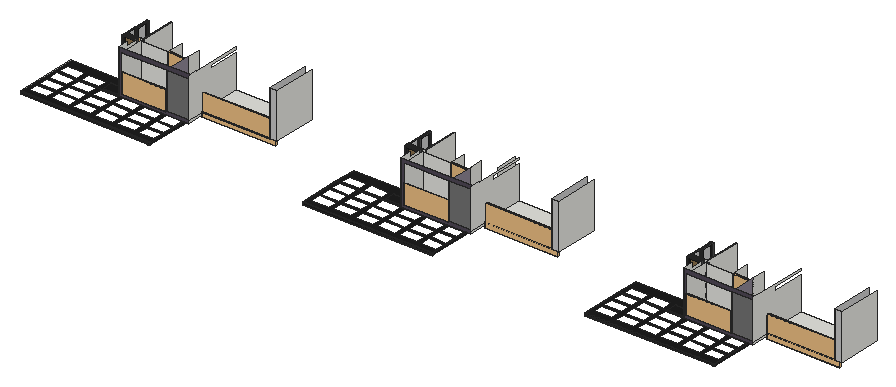
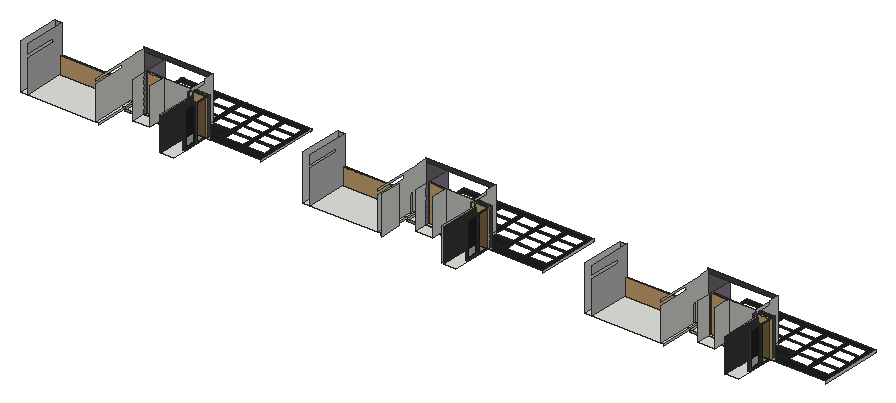
# SketchUp Ruby script. Lengths in inches.
U = 1.inch
M = Sketchup.active_model
def pt(a) = Geom::Point3d.new(a.map { |v| v * U })
def face(e, loops, mat)
  f = e.add_face(loops[0].map { |a| pt(a) })
  loops[1..].each { |l| e.add_face(l.map { |a| pt(a) }).erase! }
  f.material = f.back_material = mat if mat
  f
end
# faces: each face lists its corners as indices into pts; further lists are holes
def faces(e, pts, list, mat = nil) = list.each { |f| face(e, (f[0].is_a?(Array) ? f : [f]).map { |l| l.map { |i| pts[i] } }, mat) }
# xy, xz, yz: faces in a plane at the given z, y or x. An outline is a flat list of corners, or four numbers for a rectangle; further outlines are holes
def ring(l) = l.size == 4 ? [[l[0], l[1]], [l[2], l[1]], [l[2], l[3]], [l[0], l[3]]] : l.each_slice(2).to_a
def flat(e, list, mat, &to3) = list.each { |f| face(e, (f[0].is_a?(Array) ? f : [f]).map { |l| ring(l).map { |u, v| to3.(u, v) } }, mat) }
def xy(e, z, list, mat = nil) = flat(e, list, mat) { |x, y| [x, y, z] }
def xz(e, y, list, mat = nil) = flat(e, list, mat) { |x, z| [x, y, z] }
def yz(e, x, list, mat = nil) = flat(e, list, mat) { |y, z| [x, y, z] }
def lines(e, pts, list) = list.each { |a, b| e.add_line(pt(pts[a]), pt(pts[b])) }
# prism: a flat outline (further loops are holes) pulled along v
def prism(e, loops, v, mat = nil)
  f = face(e, loops, mat); d = Geom::Vector3d.new(v.map { |x| x * U })
  f.pushpull(f.normal.samedirection?(d) ? d.length : -d.length)
end
def box(e, o, s, mat = nil) = prism(e, [[o, [o[0] + s[0], o[1], o[2]], [o[0] + s[0], o[1] + s[1], o[2]], [o[0], o[1] + s[1], o[2]]]], [0, 0, s[2]], mat)
def at(x, y, z, deg = 0) = Geom::Transformation.translation(pt([x, y, z])) * Geom::Transformation.rotation(ORIGIN, Z_AXIS, deg.degrees)
def axes(o, x, y, z) = Geom::Transformation.new([*x, 0, *y, 0, *z, 0, *pt(o).to_a, 1])
def part(name) = M.definitions.add(name)
# library, detail: a bought-in or finely detailed component or shape, given as its bounding box
def library(name, o, s) = part(name).tap { |d| box(d.entities, o, s) }
def detail(e, o, s) = box(e.add_group.entities, o, s)
def put(e, d, t, mat = nil) = e.add_instance(d, t).tap { |i| i.material = mat if mat }
def group(e, t, mat = nil) = e.add_group.tap { |g| g.transformation = t; g.material = mat if mat }.entities
root = M.entities
M.materials.add("Glass_Tinted_Gray").color = [0, 0, 0]
M.materials["Glass_Tinted_Gray"].alpha = 0.125
M.materials.add("[0135_DarkGray]").color = [81, 81, 81]
M.materials.add("[Color M02]").color = [198, 198, 198]
M.materials.add("[Color M04]").color = [60, 133, 34]
M.materials.add("[Color M05]1").color = [114, 114, 114]
M.materials.add("[Color M06]").color = [79, 71, 84]
M.materials.add("[Color M07]").color = [58, 58, 58]
M.materials.add("[Color M08]").color = [30, 30, 30]
M.materials.add("[Formica Graystone]1").color = [140, 132, 147]
M.materials.add("[Mirror 02]").color = [229, 229, 229]
c1 = part("glass-railing")
detail(c1.entities,[0,0,0],[1.26,75.59,33.1875])
c2 = library("Sliding Gate",[0,0,0],[194.88,4.13,70.58])
c3 = part("PENTEK_RP Fineline 50S_SlidingDoor_Glass")
box(c3.entities,[0,0,0],[46.58,0.16,94.39],"Glass_Tinted_Gray")
c4 = part("PENTEK_RP Fineline 50S_SlidingDoor_GlazingBead")
box(c4.entities,[0,0,0],[45.47,0.59,0.56],"[0135_DarkGray]")
c5 = part("PENTEK_RP Fineline 50S_SlidingDoor_GlazingBead_2")
box(c5.entities,[0,0,0],[0.56,0.59,94.39],"[0135_DarkGray]")
c6 = part("PENTEK_RP Fineline 50S_SlidingDoor_Leaf_E1")
xy(c6.entities,0,[[0,0,0.93,1.97],[0.93,1.57,1.49,1.97]],"[0135_DarkGray]")
xy(c6.entities,96.25,[[0,0,0.93,0,0.93,1.57,1.49,1.57,1.49,1.97,0,1.97]],"[0135_DarkGray]")
xz(c6.entities,0,[[0,0,0.93,96.25]],"[0135_DarkGray]")
xz(c6.entities,1.57,[[0.93,0,1.49,95.32],[0.93,95.32,1.49,96.25]],"[0135_DarkGray]")
xz(c6.entities,1.97,[[0,0,1.49,96.25]],"[0135_DarkGray]")
yz(c6.entities,0,[[0,0,1.97,96.25]],"[0135_DarkGray]")
yz(c6.entities,0.93,[[0,0,1.57,0.93],[0,0.93,1.57,95.32],[0,95.32,1.57,96.25]],"[0135_DarkGray]")
yz(c6.entities,1.49,[[1.57,0,1.97,95.32],[1.57,95.32,1.97,96.25]],"[0135_DarkGray]")
c7 = part("PENTEK_RP Fineline 50S_SlidingDoor_Leaf_E2")
xy(c7.entities,0,[[0,0,0,1.57,0.56,1.57,0.56,1.97,46.02,1.97,46.02,1.57,46.58,1.57,46.58,0]],"[0135_DarkGray]")
xy(c7.entities,0.93,[[0,0,46.58,1.57]],"[0135_DarkGray]")
xy(c7.entities,1.49,[[0.56,1.57,46.02,1.97]],"[0135_DarkGray]")
xz(c7.entities,0,[[0,0,46.58,0.93]],"[0135_DarkGray]")
xz(c7.entities,1.57,[[0,0,0.56,0.93],[46.02,0,46.58,0.93],[0.56,0.93,46.02,1.49]],"[0135_DarkGray]")
xz(c7.entities,1.97,[[0.56,0,46.02,1.49]],"[0135_DarkGray]")
yz(c7.entities,0,[[0,0,1.57,0.93]],"[0135_DarkGray]")
yz(c7.entities,0.56,[[1.57,0,1.97,0.93],[1.57,0.93,1.97,1.49]],"[0135_DarkGray]")
yz(c7.entities,46.02,[[1.57,0,1.97,0.93],[1.57,0.93,1.97,1.49]],"[0135_DarkGray]")
yz(c7.entities,46.58,[[0,0,1.57,0.93]],"[0135_DarkGray]")
c8 = part("PENTEK_RP Fineline 50S_SlidingDoor_Leaf2")
put(c8.entities,c3,at(1.49,1.42,0.93))
put(c8.entities,c4,at(1.49,0,94.77))
put(c8.entities,c5,at(46.96,0,0.93))
put(c8.entities,c3,at(1.49,0.59,0.93),"[Mirror 02]")
put(c8.entities,c5,at(0.93,0,0.93))
put(c8.entities,c6,at(0,0,0))
put(c8.entities,c6,axes([48.44,0,0],[-1,0,0],[0,1,0],[0,0,1]))
put(c8.entities,c4,at(1.49,0,0.93))
put(c8.entities,c7,axes([0.93,0,96.25],[1,0,0],[0,1,0],[0,0,-1]))
put(c8.entities,c7,at(0.93,0,0))
c9 = library("Aluprof_MB-86_Drzwi_panelowe_003_S-0452",[0,0,0],[44.84,5.36,87])
c10 = library("Group\#1",[0,0,0],[29.75,5.78,110.95])
xy(root,117.06,[[264.14,305.5,671.22,306.625],[1150.61,305.5,1557.68,306.625],[2037.07,305.5,2444.15,306.625],[670.9,306.625,671.22,487.3125],[1557.37,306.625,1557.68,487.3125],
  [2443.83,306.625,2444.15,487.3125]])
xy(root,123.92,[[618.43,305.5,671.22,306.625],[1504.89,305.5,1557.68,306.625],[2391.36,305.5,2444.15,306.625],[670.9,306.625,671.22,487.3125],[1557.37,306.625,1557.68,487.3125],
  [2443.83,306.625,2444.15,487.3125]])
xy(root,123.92,[[264.14,305.5,473.73,306.625],[473.73,305.5,618.43,306.625],[1150.61,305.5,1360.2,306.625],[1360.2,305.5,1504.89,306.625],[2037.07,305.5,2246.66,306.625],
  [2246.66,305.5,2391.36,306.625]],"[Color M08]")
xy(root,125.0625,[[468.02,437.0625,468.02,441.875,470.84,441.875,470.84,475.3125,468.02,475.3125,468.02,521.5625,473.73,521.5625,473.73,437.0625],[[473.73,437.0625,618.43,521.5625],[481.77,441.875,539.73,475.3125],[550.67,442.1875,608.63,475.3125]],[[618.43,437.0625,618.43,521.5625,677.53,521.5625,677.53,487.3125,671.22,487.3125,671.22,437.0625],[619.57,441.86,669.03,475.3125]],[671.22,437.0625,686.84,487.3125],[1354.48,437.0625,1354.48,441.875,1357.3,441.875,1357.3,475.3125,1354.48,475.3125,1354.48,521.5625,1360.2,521.5625,1360.2,437.0625],
  [[1360.2,437.0625,1504.89,521.5625],[1368.24,441.875,1426.2,475.3125],[1437.14,442.1875,1495.1,475.3125]],[[1504.89,437.0625,1504.89,521.5625,1563.99,521.5625,1563.99,487.3125,1557.68,487.3125,1557.68,437.0625],[1506.03,441.86,1555.49,475.3125]],[1557.68,437.0625,1573.31,487.3125],[2240.94,437.0625,2240.94,441.875,2243.76,441.875,2243.76,475.3125,2240.94,475.3125,2240.94,521.5625,2246.66,521.5625,2246.66,437.0625],[[2246.66,437.0625,2391.36,521.5625],[2254.7,441.875,2312.66,475.3125],[2323.6,442.1875,2381.56,475.3125]],
  [[2391.36,437.0625,2391.36,521.5625,2450.46,521.5625,2450.46,487.3125,2444.15,487.3125,2444.15,437.0625],[2392.5,441.86,2441.96,475.3125]],[2444.15,437.0625,2459.77,487.3125],[468.02,441.875,470.84,475.3125],[1354.48,441.875,1357.3,475.3125],[2240.94,441.875,2243.76,475.3125]])
xy(root,125.0625,[[[264.14,305.5,671.22,437.0625],[412.875,401.625,470.84,435.86],[481.77,401.625,539.73,435.86],[343.98,401.625,401.9375,435.86],[550.67,401.75,608.63,435.86],[412.875,362.375,470.84,396.41],[481.77,362.375,539.73,396.41],[343.98,362.375,401.9375,396.41],[275.89,401.625,333.04,435.86],[275.89,362.375,333.04,396.41],[550.67,362.875,608.63,396.41],[412.875,323.5,470.84,356.95],[481.77,323.5,539.73,356.95],[550.67,323.5,608.63,356.95],[343.98,323.5,401.9375,356.95],[275.89,323.5,333.04,356.95],[619.57,402.41,669.03,435.86],[619.57,362.95,669.03,396.41],[619.57,323.5,669.03,356.95]],[[1150.61,305.5,1557.68,437.0625],[1368.24,401.625,1426.2,435.86],[1230.44,401.625,1288.4,435.86],[1299.34,401.625,1357.3,435.86],[1437.14,401.75,1495.1,435.86],[1368.24,362.375,1426.2,396.41],[1230.44,362.375,1288.4,396.41],[1299.34,362.375,1357.3,396.41],[1162.36,401.625,1219.5,435.86],[1162.36,362.375,1219.5,396.41],[1437.14,362.875,1495.1,396.41],[1368.24,323.5,1426.2,356.95],[1437.14,323.5,1495.1,356.95],[1230.44,323.5,1288.4,356.95],[1299.34,323.5,1357.3,356.95],[1162.36,323.5,1219.5,356.95],[1506.03,402.41,1555.49,435.86],[1506.03,362.95,1555.49,396.41],[1506.03,323.5,1555.49,356.95]],[[2037.07,305.5,2444.15,437.0625],[2185.8,401.625,2243.76,435.86],[2254.7,401.625,2312.66,435.86],[2116.91,401.625,2174.87,435.86],[2323.6,401.75,2381.56,435.86],[2185.8,362.375,2243.76,396.41],[2254.7,362.375,2312.66,396.41],[2116.91,362.375,2174.87,396.41],[2048.82,401.625,2105.97,435.86],[2048.82,362.375,2105.97,396.41],[2323.6,362.875,2381.56,396.41],[2185.8,323.5,2243.76,356.95],[2254.7,323.5,2312.66,356.95],[2323.6,323.5,2381.56,356.95],[2116.91,323.5,2174.87,356.95],[2048.82,323.5,2105.97,356.95],[2392.5,402.41,2441.96,435.86],[2392.5,362.95,2441.96,396.41],[2392.5,323.5,2441.96,356.95]],[[264.14,437.0625,468.02,437.0625,468.02,441.875,412.875,441.875,412.875,475.3125,468.02,475.3125,468.02,505.3125,264.14,505.3125],[343.98,441.875,401.9375,475.3125],[275.89,441.875,333.04,475.3125]],[[1150.61,437.0625,1354.48,437.0625,1354.48,441.875,1299.34,441.875,1299.34,475.3125,1354.48,475.3125,1354.48,505.3125,1150.61,505.3125],[1230.44,441.875,1288.4,475.3125],[1162.36,441.875,1219.5,475.3125]],
  [[2037.07,437.0625,2240.94,437.0625,2240.94,441.875,2185.8,441.875,2185.8,475.3125,2240.94,475.3125,2240.94,505.3125,2037.07,505.3125],[2116.91,441.875,2174.87,475.3125],[2048.82,441.875,2105.97,475.3125]],[412.875,441.875,468.02,475.3125],[1299.34,441.875,1354.48,475.3125],[2185.8,441.875,2240.94,475.3125]],"[Color M08]")
xy(root,131.0625,[[435.78,561.375,446.59,562.32],[1322.24,561.375,1333.06,562.32],[2208.71,561.375,2219.52,562.32]])
xy(root,135.875,[[478.55,437.0625,618.43,437.0625,618.43,521.5625,565.03,521.5625,565.03,509.6875,478.55,509.6875],[1365.01,437.0625,1504.89,437.0625,1504.89,521.5625,1451.49,521.5625,1451.49,509.6875,1365.01,509.6875],[2251.48,437.0625,2391.36,437.0625,2391.36,521.5625,2337.96,521.5625,2337.96,509.6875,2251.48,509.6875],[478.55,509.6875,565.03,521.5625],[1365.01,509.6875,1451.49,521.5625],
  [2251.48,509.6875,2337.96,521.5625],[565.03,521.5625,618.43,562.32],[1451.49,521.5625,1504.89,562.32],[2337.96,521.5625,2391.36,562.32]])
xy(root,136.125,[[677.53,487.3125,686.84,521.5625],[686.84,487.3125,901.22,623.84],[901.22,487.3125,923.77,623.84],[1563.99,487.3125,1573.31,521.5625],[1573.31,487.3125,1787.6875,623.84],
  [1787.6875,487.3125,1810.23,623.84],[2450.46,487.3125,2459.77,521.5625],[2459.77,487.3125,2674.15,623.84],[2674.15,487.3125,2696.7,623.84],[424.39,505.3125,463.64,646.3125],
  [463.64,505.3125,468.02,562.32],[1310.86,505.3125,1350.1,646.3125],[1350.1,505.3125,1354.48,562.32],[2197.32,505.3125,2236.57,646.3125],[2236.57,505.3125,2240.94,562.32],
  [677.53,521.5625,686.84,623.84],[1563.99,521.5625,1573.31,623.84],[2450.46,521.5625,2459.77,623.84],[463.64,562.32,468.02,591.8125],[468.02,562.32,478.78,591.8125],
  [1350.1,562.32,1354.48,591.8125],[1354.48,562.32,1365.24,591.8125],[2236.57,562.32,2240.94,591.8125],[2240.94,562.32,2251.71,591.8125]])
xz(root,305.5,[[264.14,123.92,671.22,125.0625],[1150.61,123.92,1557.68,125.0625],[2037.07,123.92,2444.15,125.0625]],"[Color M08]")
xz(root,306.625,[[264.14,117.06,670.9,123.92],[1150.61,117.06,1557.37,123.92],[2037.07,117.06,2443.83,123.92]],"[Color M08]")
xz(root,437.0625,[[618.43,135.875,686.84,251.0625],[1504.89,135.875,1573.31,251.0625],[2391.36,135.875,2459.77,251.0625]],"[Color M05]1")
xz(root,437.0625,[[468.02,125.0625,686.84,125.0625,686.84,135.875,478.55,135.875,478.55,250.875,618.43,250.875,618.43,251.0625,686.84,251.0625,686.84,263.89,468.02,263.89],[1354.48,125.0625,1573.31,125.0625,1573.31,135.875,1365.01,135.875,1365.01,250.875,1504.89,250.875,1504.89,251.0625,1573.31,251.0625,1573.31,263.89,1354.48,263.89],[2240.94,125.0625,2459.77,125.0625,2459.77,135.875,2251.48,135.875,2251.48,250.875,2391.36,250.875,2391.36,251.0625,2459.77,251.0625,2459.77,263.89,2240.94,263.89]],"[Color M06]")
xz(root,487.3125,[[677.53,125.0625,686.84,131.0625],[1563.99,125.0625,1573.31,131.0625],[2450.46,125.0625,2459.77,131.0625],[677.53,131.0625,686.84,136.125],[1563.99,131.0625,1573.31,136.125],
  [2450.46,131.0625,2459.77,136.125]])
xz(root,487.3125,[[901.22,136.125,923.77,278.1875],[1787.6875,136.125,1810.23,278.1875],[2674.15,136.125,2696.7,278.1875]],"[Color M02]")
xz(root,505.3125,[[424.39,125.0625,468.02,136.125],[1310.86,125.0625,1354.48,136.125],[2197.32,125.0625,2240.94,136.125],[463.64,136.125,468.02,240.47],[1350.1,136.125,1354.48,240.47],
  [2236.57,136.125,2240.94,240.47]])
xz(root,509.6875,[[478.55,135.875,565.03,250.875],[1365.01,135.875,1451.49,250.875],[2251.48,135.875,2337.96,250.875]])
xz(root,521.5625,[[468.02,125.0625,473.73,131.0625],[473.73,125.0625,618.43,131.0625],[618.43,125.0625,677.53,131.0625],[1354.48,125.0625,1360.2,131.0625],[1360.2,125.0625,1504.89,131.0625],
  [1504.89,125.0625,1563.99,131.0625],[2240.94,125.0625,2246.66,131.0625],[2246.66,125.0625,2391.36,131.0625],[2391.36,125.0625,2450.46,131.0625],[468.02,131.0625,473.73,251.0625],
  [473.73,131.0625,478.55,246.25],[478.55,131.0625,618.43,135.875],[1354.48,131.0625,1360.2,251.0625],[1360.2,131.0625,1365.01,246.25],[1365.01,131.0625,1504.89,135.875],
  [2240.94,131.0625,2246.66,251.0625],[2246.66,131.0625,2251.48,246.25],[2251.48,131.0625,2391.36,135.875]])
yz(root,264.14,[[305.5,117.06,306.625,117.65],[305.5,117.65,306.625,123.92],[306.625,117.65,306.625,123.92,305.5,123.92,305.5,125.0625,505.3125,125.0625,505.3125,117.65]])
yz(root,435.78,[[561.375,131.0625,562.32,136.125]])
yz(root,463.64,[[505.3125,136.125,646.3125,240.47]],"[Color M07]")
yz(root,468.02,[[437.0625,125.0625,505.3125,131.0625],[505.3125,125.0625,521.5625,136.125],[437.0625,131.0625,437.0625,263.89,469.875,263.89,469.875,251.0625,505.3125,251.0625,505.3125,131.0625],[505.3125,136.125,521.5625,240.47],[521.5625,136.125,646.3125,240.47]])
yz(root,478.55,[[437.0625,135.875,509.6875,250.875],[509.6875,135.875,521.5625,246.25]])
yz(root,565.03,[[509.6875,135.875,562.32,135.875,562.32,251.0625,521.5625,251.0625,521.5625,250.875,509.6875,250.875]])
yz(root,618.43,[[521.5625,135.875,562.32,251.0625]])
yz(root,618.43,[[437.0625,135.875,521.5625,250.875]],"[Formica Graystone]1")
yz(root,670.9,[[306.625,117.06,487.3125,123.92]],"[Color M08]")
yz(root,671.22,[[305.5,123.92,487.3125,125.0625]],"[Color M08]")
yz(root,677.53,[[487.3125,125.0625,521.5625,131.0625],[487.3125,131.0625,521.5625,136.125],[521.5625,131.0625,623.84,136.125]])
yz(root,686.84,[[437.0625,125.0625,487.3125,131.0625],[437.0625,131.0625,487.3125,131.0625,487.3125,136.125,623.84,136.125,623.84,240.88,521.5625,240.88,521.5625,242.34,522.8125,242.34,522.8125,249.61,521.5625,249.61,521.5625,251.0625,623.84,251.0625,623.84,257.0625,467.1875,257.0625,467.1875,258.95,437.0625,258.95]])
yz(root,901.22,[[487.3125,136.125,487.3125,278.1875,623.84,278.1875,623.84,251.0625,521.5625,251.0625,521.5625,249.61,522.8125,249.61,522.8125,242.34,521.5625,242.34,521.5625,240.88,623.84,240.88,623.84,136.125]],"[Color M02]")
yz(root,923.77,[[487.3125,136.125,623.84,278.1875]])
yz(root,1150.61,[[305.5,117.06,306.625,117.65],[305.5,117.65,306.625,123.92],[306.625,117.65,306.625,123.92,305.5,123.92,305.5,125.0625,505.3125,125.0625,505.3125,117.65]])
yz(root,1322.24,[[561.375,131.0625,562.32,136.125]])
yz(root,1350.1,[[505.3125,136.125,646.3125,240.47]],"[Color M07]")
yz(root,1354.48,[[437.0625,125.0625,505.3125,131.0625],[505.3125,125.0625,521.5625,136.125],[437.0625,131.0625,437.0625,263.89,469.875,263.89,469.875,251.0625,505.3125,251.0625,505.3125,131.0625],[505.3125,136.125,521.5625,240.47],[521.5625,136.125,646.3125,240.47]])
yz(root,1365.01,[[437.0625,135.875,509.6875,250.875],[509.6875,135.875,521.5625,246.25]])
yz(root,1451.49,[[509.6875,135.875,562.32,135.875,562.32,251.0625,521.5625,251.0625,521.5625,250.875,509.6875,250.875]])
yz(root,1504.89,[[521.5625,135.875,562.32,251.0625]])
yz(root,1504.89,[[437.0625,135.875,521.5625,250.875]],"[Formica Graystone]1")
yz(root,1557.37,[[306.625,117.06,487.3125,123.92]],"[Color M08]")
yz(root,1557.68,[[305.5,123.92,487.3125,125.0625]],"[Color M08]")
yz(root,1557.79,[[562.32,131.0625,630.04,251.0625]])
yz(root,1563.99,[[487.3125,125.0625,521.5625,131.0625],[487.3125,131.0625,521.5625,136.125],[521.5625,131.0625,623.84,136.125]])
yz(root,1573.31,[[437.0625,125.0625,487.3125,131.0625],[437.0625,131.0625,487.3125,131.0625,487.3125,136.125,623.84,136.125,623.84,240.88,521.5625,240.88,521.5625,242.34,522.8125,242.34,522.8125,249.61,521.5625,249.61,521.5625,251.0625,623.84,251.0625,623.84,257.0625,467.1875,257.0625,467.1875,258.95,437.0625,258.95]])
yz(root,1787.6875,[[487.3125,136.125,487.3125,278.1875,623.84,278.1875,623.84,251.0625,521.5625,251.0625,521.5625,249.61,522.8125,249.61,522.8125,242.34,521.5625,242.34,521.5625,240.88,623.84,240.88,623.84,136.125]],"[Color M02]")
yz(root,1810.23,[[487.3125,136.125,623.84,278.1875]])
yz(root,2037.07,[[305.5,117.06,306.625,117.65],[305.5,117.65,306.625,123.92],[306.625,117.65,306.625,123.92,305.5,123.92,305.5,125.0625,505.3125,125.0625,505.3125,117.65]])
yz(root,2208.71,[[561.375,131.0625,562.32,136.125]])
yz(root,2236.57,[[505.3125,136.125,646.3125,240.47]],"[Color M07]")
yz(root,2240.94,[[437.0625,125.0625,505.3125,131.0625],[505.3125,125.0625,521.5625,136.125],[437.0625,131.0625,437.0625,263.89,469.875,263.89,469.875,251.0625,505.3125,251.0625,505.3125,131.0625],[505.3125,136.125,521.5625,240.47],[521.5625,136.125,646.3125,240.47]])
yz(root,2251.48,[[437.0625,135.875,509.6875,250.875],[509.6875,135.875,521.5625,246.25]])
yz(root,2337.96,[[509.6875,135.875,562.32,135.875,562.32,251.0625,521.5625,251.0625,521.5625,250.875,509.6875,250.875]])
yz(root,2391.36,[[521.5625,135.875,562.32,251.0625]])
yz(root,2391.36,[[437.0625,135.875,521.5625,250.875]],"[Formica Graystone]1")
yz(root,2443.83,[[306.625,117.06,487.3125,123.92]],"[Color M08]")
yz(root,2444.15,[[305.5,123.92,487.3125,125.0625]],"[Color M08]")
yz(root,2450.46,[[487.3125,125.0625,521.5625,131.0625],[487.3125,131.0625,521.5625,136.125],[521.5625,131.0625,623.84,136.125]])
yz(root,2459.77,[[437.0625,125.0625,487.3125,131.0625],[437.0625,131.0625,487.3125,131.0625,487.3125,136.125,623.84,136.125,623.84,240.88,521.5625,240.88,521.5625,242.34,522.8125,242.34,522.8125,249.61,521.5625,249.61,521.5625,251.0625,623.84,251.0625,623.84,257.0625,467.1875,257.0625,467.1875,258.95,437.0625,258.95]])
yz(root,2674.15,[[487.3125,136.125,487.3125,278.1875,623.84,278.1875,623.84,251.0625,521.5625,251.0625,521.5625,249.61,522.8125,249.61,522.8125,242.34,521.5625,242.34,521.5625,240.88,623.84,240.88,623.84,136.125]],"[Color M02]")
yz(root,2696.7,[[487.3125,136.125,623.84,278.1875]])
p = [[1360.2,521.5625,131.0625],[1360.2,467.1875,131.0625],[1365.01,521.5625,131.0625],[1365.01,467.1875,131.0625],[1316.04,521.5625,131.0625],[1316.04,521.5625,136.125],
  [2246.66,521.5625,131.0625],[2246.66,467.1875,131.0625],[2202.51,521.5625,131.0625],[2202.51,521.5625,136.125],[2251.48,521.5625,131.0625],[2251.48,467.1875,131.0625],
  [478.55,521.5625,131.0625],[478.55,467.1875,131.0625],[429.58,521.5625,131.0625],[429.58,521.5625,136.125],[473.73,521.5625,131.0625],[473.73,467.1875,131.0625]]
lines(root,p,[[0,1],[2,3],[4,5],[6,7],[8,9],[10,11],[12,13],[14,15],[16,17]])
put(root,c1,axes([1365.01,437.0625,135.875],[0,-1.85,0],[1.85,0,0],[0,0,1.85]))
put(root,c1,axes([2251.48,437.0625,135.875],[0,-1.85,0],[1.85,0,0],[0,0,1.85]))
put(root,c1,axes([478.55,437.0625,135.875],[0,-1.85,0],[1.85,0,0],[0,0,1.85]))
put(root,c2,axes([1573.31,491.03,118.7],[1.17982,0,0],[0,1,0],[0,0,1]))
put(root,c2,axes([2459.77,491.03,118.7],[1.17982,0,0],[0,1,0],[0,0,1]))
put(root,c2,axes([686.84,491.03,118.7],[1.17982,0,0],[0,1,0],[0,0,1]))
put(root,c8,axes([1310.86,505.3125,136.125],[0.90045,0,0],[0,3.85,0],[0,0,1.1941]))
put(root,c8,axes([2197.32,505.3125,136.125],[0.90045,0,0],[0,3.85,0],[0,0,1.1941]))
put(root,c8,axes([424.39,505.3125,136.125],[0.90045,0,0],[0,3.85,0],[0,0,1.1941]))
put(root,c9,axes([1451.49,508.78,135.875],[1.16659,-0.08923,0],[0.08923,1.16659,0],[0,0,1.32399]))
put(root,c9,axes([2337.96,508.78,135.875],[1.16659,-0.08923,0],[0.08923,1.16659,0],[0,0,1.32399]))
put(root,c9,axes([565.03,508.78,135.875],[1.16659,-0.08923,0],[0.08923,1.16659,0],[0,0,1.32399]))
put(root,c10,axes([1310.86,515.625,136.125],[1.38276,0,0],[0,1,0],[0,0,1.03593]),"[Color M04]")
put(root,c10,axes([2197.32,515.625,136.125],[1.38276,0,0],[0,1,0],[0,0,1.03593]),"[Color M04]")
put(root,c10,axes([424.39,515.625,136.125],[1.38276,0,0],[0,1,0],[0,0,1.03593]),"[Color M04]")
put(root,c8,axes([1310.87,556.51,136.125],[0,-0.90045,0],[0.924,0,0],[0,0,1.1941]))
put(root,c8,axes([2197.33,556.51,136.125],[0,-0.90045,0],[0.924,0,0],[0,0,1.1941]))
put(root,c8,axes([424.4,556.51,136.125],[0,-0.90045,0],[0.924,0,0],[0,0,1.1941]))
put(root,c8,axes([1310.86,600.14,136.125],[0,-0.90045,0],[3.85,0,0],[0,0,1.1941]))
put(root,c8,axes([2197.32,600.14,136.125],[0,-0.90045,0],[3.85,0,0],[0,0,1.1941]))
put(root,c8,axes([424.39,600.14,136.125],[0,-0.90045,0],[3.85,0,0],[0,0,1.1941]))
